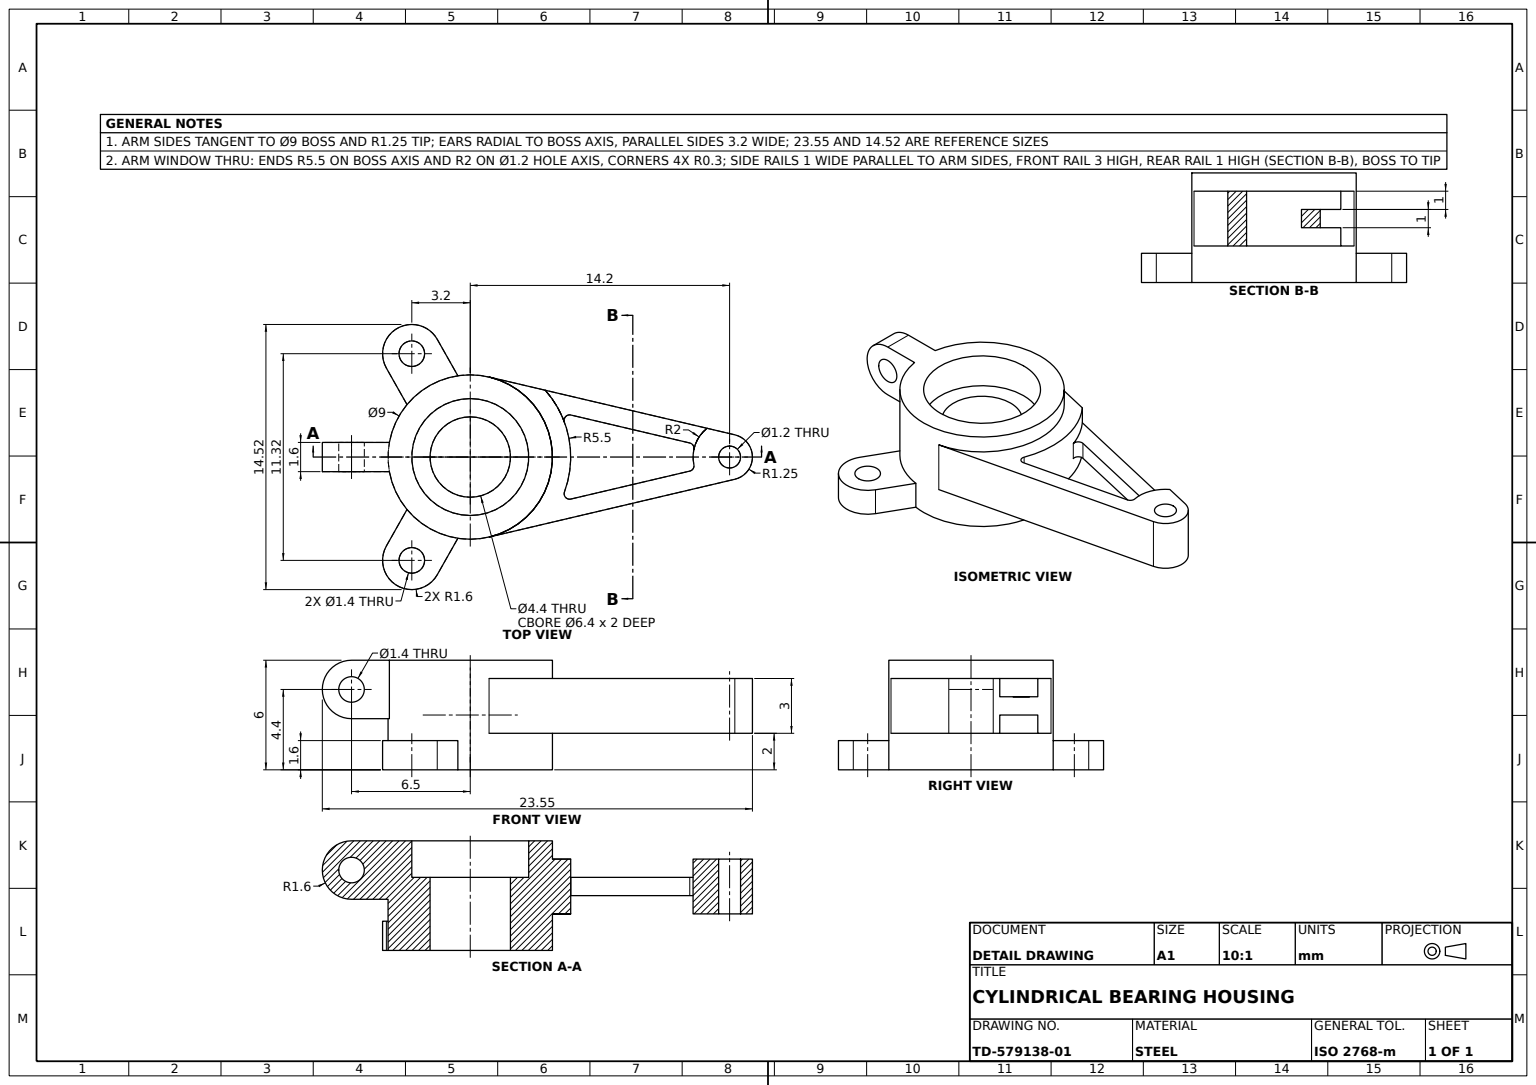
ISO-10303-21;
HEADER;
FILE_DESCRIPTION((''),'2;1');
FILE_NAME('','',(''),(''),'','','');
FILE_SCHEMA(('AUTOMOTIVE_DESIGN'));
ENDSEC;
DATA;
#1=APPLICATION_CONTEXT('');
#2=PRODUCT_CONTEXT('',#1,'mechanical');
#3=PRODUCT('','','',(#2));
#4=PRODUCT_DEFINITION_FORMATION('','',#3);
#5=PRODUCT_DEFINITION_CONTEXT('',#1,'design');
#6=PRODUCT_DEFINITION('','',#4,#5);
#7=PRODUCT_DEFINITION_SHAPE('','',#6);
#8=(LENGTH_UNIT()NAMED_UNIT(*)SI_UNIT(.MILLI.,.METRE.));
#9=(NAMED_UNIT(*)PLANE_ANGLE_UNIT()SI_UNIT($,.RADIAN.));
#10=(NAMED_UNIT(*)SI_UNIT($,.STERADIAN.)SOLID_ANGLE_UNIT());
#11=UNCERTAINTY_MEASURE_WITH_UNIT(LENGTH_MEASURE(1.E-05),#8,'distance_accuracy_value','');
#12=(GEOMETRIC_REPRESENTATION_CONTEXT(3)GLOBAL_UNCERTAINTY_ASSIGNED_CONTEXT((#11))GLOBAL_UNIT_ASSIGNED_CONTEXT((#8,#9,#10))REPRESENTATION_CONTEXT('',''));
#13=CARTESIAN_POINT('',(-3.2,1.6,-6.35773806));
#14=VERTEX_POINT('',#13);
#15=CARTESIAN_POINT('',(-3.2,1.6,-4.95773806));
#16=VERTEX_POINT('',#15);
#17=CARTESIAN_POINT('',(-3.2,1.6,-5.65773806));
#18=DIRECTION('',(0.,-1.,0.));
#19=DIRECTION('',(0.,0.,-1.));
#20=AXIS2_PLACEMENT_3D('',#17,#18,#19);
#21=CIRCLE('',#20,0.7);
#22=EDGE_CURVE('',#14,#16,#21,.T.);
#23=ORIENTED_EDGE('',*,*,#22,.T.);
#24=EDGE_CURVE('',#16,#14,#21,.T.);
#25=ORIENTED_EDGE('',*,*,#24,.T.);
#26=EDGE_LOOP('',(#23,#25));
#27=FACE_BOUND('',#26,.T.);
#28=CARTESIAN_POINT('',(-0.67794665,1.6,-4.44863893));
#29=VERTEX_POINT('',#28);
#30=CARTESIAN_POINT('',(-3.46329462,1.6,-2.87325432));
#31=VERTEX_POINT('',#30);
#32=CARTESIAN_POINT('',(0.,1.6,0.));
#33=DIRECTION('',(0.,1.,0.));
#34=AXIS2_PLACEMENT_3D('',#32,#33,#19);
#35=CIRCLE('',#34,4.5);
#36=EDGE_CURVE('',#29,#31,#35,.T.);
#37=ORIENTED_EDGE('',*,*,#36,.F.);
#38=CARTESIAN_POINT('',(-1.80732602,1.6,-6.44543037));
#39=VERTEX_POINT('',#38);
#40=DIRECTION('',(0.492307692,0.,0.870421241));
#41=VECTOR('',#40,1000.);
#42=LINE('',#28,#41);
#43=EDGE_CURVE('',#39,#29,#42,.T.);
#44=ORIENTED_EDGE('',*,*,#43,.F.);
#45=CARTESIAN_POINT('',(-3.2,1.6,-7.25773806));
#46=VERTEX_POINT('',#45);
#47=DIRECTION('',(0.,0.,1.));
#48=AXIS2_PLACEMENT_3D('',#17,#18,#47);
#49=CIRCLE('',#48,1.6);
#50=EDGE_CURVE('',#46,#39,#49,.T.);
#51=ORIENTED_EDGE('',*,*,#50,.F.);
#52=CARTESIAN_POINT('',(-4.59267398,1.6,-4.87004576));
#53=VERTEX_POINT('',#52);
#54=EDGE_CURVE('',#53,#46,#49,.T.);
#55=ORIENTED_EDGE('',*,*,#54,.F.);
#56=DIRECTION('',(-0.492307692,0.,-0.870421241));
#57=VECTOR('',#56,1000.);
#58=LINE('',#30,#57);
#59=EDGE_CURVE('',#31,#53,#58,.T.);
#60=ORIENTED_EDGE('',*,*,#59,.F.);
#61=EDGE_LOOP('',(#37,#44,#51,#55,#60));
#62=FACE_OUTER_BOUND('',#61,.T.);
#63=AXIS2_PLACEMENT_3D('',#17,#33,#47);
#64=PLANE('',#63);
#65=ADVANCED_FACE('',(#27,#62),#64,.T.);
#66=CARTESIAN_POINT('',(-3.46329462,1.6,2.87325432));
#67=VERTEX_POINT('',#66);
#68=CARTESIAN_POINT('',(-0.67794665,1.6,4.44863893));
#69=VERTEX_POINT('',#68);
#70=EDGE_CURVE('',#67,#69,#35,.T.);
#71=ORIENTED_EDGE('',*,*,#70,.T.);
#72=CARTESIAN_POINT('',(-0.67794665,0.,4.44863893));
#73=VERTEX_POINT('',#72);
#74=VECTOR('',#18,1000.);
#75=LINE('',#68,#74);
#76=EDGE_CURVE('',#69,#73,#75,.T.);
#77=ORIENTED_EDGE('',*,*,#76,.T.);
#78=CARTESIAN_POINT('',(0.,0.,4.5));
#79=VERTEX_POINT('',#78);
#80=CARTESIAN_POINT('',(0.,0.,0.));
#81=AXIS2_PLACEMENT_3D('',#80,#33,#47);
#82=CIRCLE('',#81,4.5);
#83=EDGE_CURVE('',#73,#79,#82,.T.);
#84=ORIENTED_EDGE('',*,*,#83,.T.);
#85=CARTESIAN_POINT('',(0.,6.,4.5));
#86=VERTEX_POINT('',#85);
#87=LINE('',#85,#74);
#88=EDGE_CURVE('',#86,#79,#87,.T.);
#89=ORIENTED_EDGE('',*,*,#88,.F.);
#90=CARTESIAN_POINT('',(-4.42831797,6.,0.8));
#91=VERTEX_POINT('',#90);
#92=CARTESIAN_POINT('',(0.,6.,0.));
#93=AXIS2_PLACEMENT_3D('',#92,#33,#47);
#94=CIRCLE('',#93,4.5);
#95=EDGE_CURVE('',#91,#86,#94,.T.);
#96=ORIENTED_EDGE('',*,*,#95,.F.);
#97=CARTESIAN_POINT('',(-4.42831797,2.8,0.8));
#98=VERTEX_POINT('',#97);
#99=VECTOR('',#33,1000.);
#100=LINE('',#90,#99);
#101=EDGE_CURVE('',#98,#91,#100,.T.);
#102=ORIENTED_EDGE('',*,*,#101,.F.);
#103=CARTESIAN_POINT('',(-4.42831797,2.8,-0.8));
#104=VERTEX_POINT('',#103);
#105=CARTESIAN_POINT('',(0.,2.8,0.));
#106=AXIS2_PLACEMENT_3D('',#105,#33,#47);
#107=CIRCLE('',#106,4.5);
#108=EDGE_CURVE('',#104,#98,#107,.T.);
#109=ORIENTED_EDGE('',*,*,#108,.F.);
#110=CARTESIAN_POINT('',(-4.42831797,6.,-0.8));
#111=VERTEX_POINT('',#110);
#112=LINE('',#110,#74);
#113=EDGE_CURVE('',#111,#104,#112,.T.);
#114=ORIENTED_EDGE('',*,*,#113,.F.);
#115=CARTESIAN_POINT('',(0.,6.,-4.5));
#116=VERTEX_POINT('',#115);
#117=EDGE_CURVE('',#116,#111,#94,.T.);
#118=ORIENTED_EDGE('',*,*,#117,.F.);
#119=CARTESIAN_POINT('',(0.,0.,-4.5));
#120=VERTEX_POINT('',#119);
#121=LINE('',#115,#74);
#122=EDGE_CURVE('',#116,#120,#121,.T.);
#123=ORIENTED_EDGE('',*,*,#122,.T.);
#124=CARTESIAN_POINT('',(-0.67794665,0.,-4.44863893));
#125=VERTEX_POINT('',#124);
#126=EDGE_CURVE('',#120,#125,#82,.T.);
#127=ORIENTED_EDGE('',*,*,#126,.T.);
#128=LINE('',#28,#74);
#129=EDGE_CURVE('',#29,#125,#128,.T.);
#130=ORIENTED_EDGE('',*,*,#129,.F.);
#131=ORIENTED_EDGE('',*,*,#36,.T.);
#132=CARTESIAN_POINT('',(-3.46329462,0.,-2.87325432));
#133=VERTEX_POINT('',#132);
#134=LINE('',#30,#74);
#135=EDGE_CURVE('',#31,#133,#134,.T.);
#136=ORIENTED_EDGE('',*,*,#135,.T.);
#137=CARTESIAN_POINT('',(-3.46329462,0.,2.87325432));
#138=VERTEX_POINT('',#137);
#139=EDGE_CURVE('',#133,#138,#82,.T.);
#140=ORIENTED_EDGE('',*,*,#139,.T.);
#141=LINE('',#66,#74);
#142=EDGE_CURVE('',#67,#138,#141,.T.);
#143=ORIENTED_EDGE('',*,*,#142,.F.);
#144=EDGE_LOOP('',(#71,#77,#84,#89,#96,#102,#109,#114,#118,#123,#127,#130,#131,#136,#140,#143));
#145=FACE_OUTER_BOUND('',#144,.T.);
#146=AXIS2_PLACEMENT_3D('',#92,#18,#19);
#147=CYLINDRICAL_SURFACE('',#146,4.5);
#148=ADVANCED_FACE('',(#145),#147,.T.);
#149=CARTESIAN_POINT('',(14.48609155,2.,1.21682029));
#150=VERTEX_POINT('',#149);
#151=CARTESIAN_POINT('',(14.48609155,2.,-1.21682029));
#152=VERTEX_POINT('',#151);
#153=CARTESIAN_POINT('',(14.2,2.,0.));
#154=AXIS2_PLACEMENT_3D('',#153,#33,#47);
#155=CIRCLE('',#154,1.25);
#156=EDGE_CURVE('',#150,#152,#155,.T.);
#157=ORIENTED_EDGE('',*,*,#156,.F.);
#158=CARTESIAN_POINT('',(1.02992958,2.,4.38055305));
#159=VERTEX_POINT('',#158);
#160=DIRECTION('',(0.973456234,0.,-0.228873239));
#161=VECTOR('',#160,1000.);
#162=LINE('',#158,#161);
#163=EDGE_CURVE('',#159,#150,#162,.T.);
#164=ORIENTED_EDGE('',*,*,#163,.F.);
#165=CARTESIAN_POINT('',(1.02992958,2.,-4.38055305));
#166=VERTEX_POINT('',#165);
#167=CARTESIAN_POINT('',(0.,2.,0.));
#168=AXIS2_PLACEMENT_3D('',#167,#18,#47);
#169=CIRCLE('',#168,4.5);
#170=EDGE_CURVE('',#166,#159,#169,.T.);
#171=ORIENTED_EDGE('',*,*,#170,.F.);
#172=CARTESIAN_POINT('',(4.10826848,2.,-3.65679232));
#173=VERTEX_POINT('',#172);
#174=DIRECTION('',(-0.973456234,0.,-0.228873239));
#175=VECTOR('',#174,1000.);
#176=LINE('',#165,#175);
#177=EDGE_CURVE('',#173,#166,#176,.T.);
#178=ORIENTED_EDGE('',*,*,#177,.F.);
#179=CARTESIAN_POINT('',(5.1598984,2.,1.90406105));
#180=VERTEX_POINT('',#179);
#181=CIRCLE('',#168,5.5);
#182=EDGE_CURVE('',#173,#180,#181,.T.);
#183=ORIENTED_EDGE('',*,*,#182,.T.);
#184=CARTESIAN_POINT('',(5.44134741,2.,2.30791892));
#185=VERTEX_POINT('',#184);
#186=CARTESIAN_POINT('',(5.44134741,2.,2.00791892));
#187=AXIS2_PLACEMENT_3D('',#186,#33,#47);
#188=CIRCLE('',#187,0.3);
#189=EDGE_CURVE('',#180,#185,#188,.T.);
#190=ORIENTED_EDGE('',*,*,#189,.T.);
#191=CARTESIAN_POINT('',(5.51000938,2.,2.29995579));
#192=VERTEX_POINT('',#191);
#193=EDGE_CURVE('',#185,#192,#188,.T.);
#194=ORIENTED_EDGE('',*,*,#193,.T.);
#195=CARTESIAN_POINT('',(12.01879809,2.,0.76964811));
#196=VERTEX_POINT('',#195);
#197=CARTESIAN_POINT('',(0.80105634,2.,3.40709682));
#198=LINE('',#197,#161);
#199=EDGE_CURVE('',#192,#196,#198,.T.);
#200=ORIENTED_EDGE('',*,*,#199,.T.);
#201=CARTESIAN_POINT('',(12.24359662,2.,0.41531412));
#202=VERTEX_POINT('',#201);
#203=CARTESIAN_POINT('',(11.95013611,2.,0.47761124));
#204=AXIS2_PLACEMENT_3D('',#203,#33,#47);
#205=CIRCLE('',#204,0.3);
#206=EDGE_CURVE('',#196,#202,#205,.T.);
#207=ORIENTED_EDGE('',*,*,#206,.T.);
#208=CARTESIAN_POINT('',(12.96628349,2.,-1.57414852));
#209=VERTEX_POINT('',#208);
#210=AXIS2_PLACEMENT_3D('',#153,#18,#47);
#211=CIRCLE('',#210,2.);
#212=EDGE_CURVE('',#202,#209,#211,.T.);
#213=ORIENTED_EDGE('',*,*,#212,.T.);
#214=EDGE_CURVE('',#152,#209,#176,.T.);
#215=ORIENTED_EDGE('',*,*,#214,.F.);
#216=EDGE_LOOP('',(#157,#164,#171,#178,#183,#190,#194,#200,#207,#213,#215));
#217=FACE_OUTER_BOUND('',#216,.T.);
#218=CARTESIAN_POINT('',(14.2,2.,0.6));
#219=VERTEX_POINT('',#218);
#220=CARTESIAN_POINT('',(14.2,2.,-0.6));
#221=VERTEX_POINT('',#220);
#222=CIRCLE('',#154,0.6);
#223=EDGE_CURVE('',#219,#221,#222,.T.);
#224=ORIENTED_EDGE('',*,*,#223,.T.);
#225=EDGE_CURVE('',#221,#219,#222,.T.);
#226=ORIENTED_EDGE('',*,*,#225,.T.);
#227=EDGE_LOOP('',(#224,#226));
#228=FACE_BOUND('',#227,.T.);
#229=AXIS2_PLACEMENT_3D('',#167,#33,#47);
#230=PLANE('',#229);
#231=ADVANCED_FACE('',(#217,#228),#230,.F.);
#232=CARTESIAN_POINT('',(-8.1,4.4,0.8));
#233=VERTEX_POINT('',#232);
#234=CARTESIAN_POINT('',(-8.1,4.4,-0.8));
#235=VERTEX_POINT('',#234);
#236=VECTOR('',#19,1000.);
#237=LINE('',#232,#236);
#238=EDGE_CURVE('',#233,#235,#237,.T.);
#239=ORIENTED_EDGE('',*,*,#238,.T.);
#240=CARTESIAN_POINT('',(-6.5,2.8,-0.8));
#241=VERTEX_POINT('',#240);
#242=CARTESIAN_POINT('',(-6.5,4.4,-0.8));
#243=DIRECTION('',(1.,0.,0.));
#244=AXIS2_PLACEMENT_3D('',#242,#47,#243);
#245=CIRCLE('',#244,1.6);
#246=EDGE_CURVE('',#235,#241,#245,.T.);
#247=ORIENTED_EDGE('',*,*,#246,.T.);
#248=CARTESIAN_POINT('',(-6.5,2.8,0.8));
#249=VERTEX_POINT('',#248);
#250=LINE('',#248,#236);
#251=EDGE_CURVE('',#249,#241,#250,.T.);
#252=ORIENTED_EDGE('',*,*,#251,.F.);
#253=CARTESIAN_POINT('',(-6.5,4.4,0.8));
#254=AXIS2_PLACEMENT_3D('',#253,#47,#243);
#255=CIRCLE('',#254,1.6);
#256=EDGE_CURVE('',#233,#249,#255,.T.);
#257=ORIENTED_EDGE('',*,*,#256,.F.);
#258=EDGE_LOOP('',(#239,#247,#252,#257));
#259=FACE_OUTER_BOUND('',#258,.T.);
#260=DIRECTION('',(-1.,0.,0.));
#261=AXIS2_PLACEMENT_3D('',#253,#19,#260);
#262=CYLINDRICAL_SURFACE('',#261,1.6);
#263=ADVANCED_FACE('',(#259),#262,.T.);
#264=CARTESIAN_POINT('',(-4.59267398,0.,-4.87004576));
#265=VERTEX_POINT('',#264);
#266=CARTESIAN_POINT('',(-3.2,0.,-7.25773806));
#267=VERTEX_POINT('',#266);
#268=CARTESIAN_POINT('',(-3.2,0.,-5.65773806));
#269=AXIS2_PLACEMENT_3D('',#268,#18,#47);
#270=CIRCLE('',#269,1.6);
#271=EDGE_CURVE('',#265,#267,#270,.T.);
#272=ORIENTED_EDGE('',*,*,#271,.F.);
#273=LINE('',#52,#74);
#274=EDGE_CURVE('',#53,#265,#273,.T.);
#275=ORIENTED_EDGE('',*,*,#274,.F.);
#276=ORIENTED_EDGE('',*,*,#54,.T.);
#277=LINE('',#45,#74);
#278=EDGE_CURVE('',#46,#267,#277,.T.);
#279=ORIENTED_EDGE('',*,*,#278,.T.);
#280=EDGE_LOOP('',(#272,#275,#276,#279));
#281=FACE_OUTER_BOUND('',#280,.T.);
#282=CYLINDRICAL_SURFACE('',#20,1.6);
#283=ADVANCED_FACE('',(#281),#282,.T.);
#284=CARTESIAN_POINT('',(0.,6.,3.2));
#285=VERTEX_POINT('',#284);
#286=CARTESIAN_POINT('',(0.,6.,-3.2));
#287=VERTEX_POINT('',#286);
#288=CIRCLE('',#93,3.2);
#289=EDGE_CURVE('',#285,#287,#288,.T.);
#290=ORIENTED_EDGE('',*,*,#289,.T.);
#291=CARTESIAN_POINT('',(0.,4.,-3.2));
#292=VERTEX_POINT('',#291);
#293=LINE('',#286,#99);
#294=EDGE_CURVE('',#292,#287,#293,.T.);
#295=ORIENTED_EDGE('',*,*,#294,.F.);
#296=CARTESIAN_POINT('',(0.,4.,3.2));
#297=VERTEX_POINT('',#296);
#298=CARTESIAN_POINT('',(0.,4.,0.));
#299=AXIS2_PLACEMENT_3D('',#298,#33,#47);
#300=CIRCLE('',#299,3.2);
#301=EDGE_CURVE('',#297,#292,#300,.T.);
#302=ORIENTED_EDGE('',*,*,#301,.F.);
#303=LINE('',#284,#99);
#304=EDGE_CURVE('',#297,#285,#303,.T.);
#305=ORIENTED_EDGE('',*,*,#304,.T.);
#306=EDGE_LOOP('',(#290,#295,#302,#305));
#307=FACE_OUTER_BOUND('',#306,.T.);
#308=CYLINDRICAL_SURFACE('',#93,3.2);
#309=ADVANCED_FACE('',(#307),#308,.F.);
#310=CARTESIAN_POINT('',(-1.80732602,1.6,6.44543037));
#311=VERTEX_POINT('',#310);
#312=CARTESIAN_POINT('',(-1.80732602,0.,6.44543037));
#313=VERTEX_POINT('',#312);
#314=LINE('',#310,#74);
#315=EDGE_CURVE('',#311,#313,#314,.T.);
#316=ORIENTED_EDGE('',*,*,#315,.F.);
#317=CARTESIAN_POINT('',(-4.59267398,1.6,4.87004576));
#318=VERTEX_POINT('',#317);
#319=CARTESIAN_POINT('',(-3.2,1.6,5.65773806));
#320=AXIS2_PLACEMENT_3D('',#319,#18,#19);
#321=CIRCLE('',#320,1.6);
#322=EDGE_CURVE('',#311,#318,#321,.T.);
#323=ORIENTED_EDGE('',*,*,#322,.T.);
#324=CARTESIAN_POINT('',(-4.59267398,0.,4.87004576));
#325=VERTEX_POINT('',#324);
#326=LINE('',#317,#74);
#327=EDGE_CURVE('',#318,#325,#326,.T.);
#328=ORIENTED_EDGE('',*,*,#327,.T.);
#329=CARTESIAN_POINT('',(-3.2,0.,5.65773806));
#330=AXIS2_PLACEMENT_3D('',#329,#18,#19);
#331=CIRCLE('',#330,1.6);
#332=EDGE_CURVE('',#313,#325,#331,.T.);
#333=ORIENTED_EDGE('',*,*,#332,.F.);
#334=EDGE_LOOP('',(#316,#323,#328,#333));
#335=FACE_OUTER_BOUND('',#334,.T.);
#336=CYLINDRICAL_SURFACE('',#320,1.6);
#337=ADVANCED_FACE('',(#335),#336,.T.);
#338=CARTESIAN_POINT('',(-7.2,4.4,0.8));
#339=VERTEX_POINT('',#338);
#340=CARTESIAN_POINT('',(-5.8,4.4,0.8));
#341=VERTEX_POINT('',#340);
#342=CIRCLE('',#254,0.7);
#343=EDGE_CURVE('',#339,#341,#342,.T.);
#344=ORIENTED_EDGE('',*,*,#343,.F.);
#345=EDGE_CURVE('',#341,#339,#342,.T.);
#346=ORIENTED_EDGE('',*,*,#345,.F.);
#347=EDGE_LOOP('',(#344,#346));
#348=FACE_BOUND('',#347,.T.);
#349=ORIENTED_EDGE('',*,*,#256,.T.);
#350=CARTESIAN_POINT('',(-3.7,2.8,0.8));
#351=VECTOR('',#260,1000.);
#352=LINE('',#350,#351);
#353=EDGE_CURVE('',#98,#249,#352,.T.);
#354=ORIENTED_EDGE('',*,*,#353,.F.);
#355=ORIENTED_EDGE('',*,*,#101,.T.);
#356=CARTESIAN_POINT('',(-6.5,6.,0.8));
#357=VERTEX_POINT('',#356);
#358=CARTESIAN_POINT('',(-3.7,6.,0.8));
#359=LINE('',#358,#351);
#360=EDGE_CURVE('',#91,#357,#359,.T.);
#361=ORIENTED_EDGE('',*,*,#360,.T.);
#362=EDGE_CURVE('',#357,#233,#255,.T.);
#363=ORIENTED_EDGE('',*,*,#362,.T.);
#364=EDGE_LOOP('',(#349,#354,#355,#361,#363));
#365=FACE_OUTER_BOUND('',#364,.T.);
#366=AXIS2_PLACEMENT_3D('',#358,#19,#260);
#367=PLANE('',#366);
#368=ADVANCED_FACE('',(#348,#365),#367,.F.);
#369=ORIENTED_EDGE('',*,*,#76,.F.);
#370=DIRECTION('',(-0.492307692,0.,0.870421241));
#371=VECTOR('',#370,1000.);
#372=LINE('',#68,#371);
#373=EDGE_CURVE('',#69,#311,#372,.T.);
#374=ORIENTED_EDGE('',*,*,#373,.T.);
#375=ORIENTED_EDGE('',*,*,#315,.T.);
#376=LINE('',#72,#371);
#377=EDGE_CURVE('',#73,#313,#376,.T.);
#378=ORIENTED_EDGE('',*,*,#377,.F.);
#379=EDGE_LOOP('',(#369,#374,#375,#378));
#380=FACE_OUTER_BOUND('',#379,.T.);
#381=DIRECTION('',(0.870421241,0.,0.492307692));
#382=DIRECTION('',(0.492307692,0.,-0.870421241));
#383=AXIS2_PLACEMENT_3D('',#68,#381,#382);
#384=PLANE('',#383);
#385=ADVANCED_FACE('',(#380),#384,.T.);
#386=CARTESIAN_POINT('',(-5.8,4.4,-0.8));
#387=VERTEX_POINT('',#386);
#388=LINE('',#340,#236);
#389=EDGE_CURVE('',#341,#387,#388,.T.);
#390=ORIENTED_EDGE('',*,*,#389,.T.);
#391=CARTESIAN_POINT('',(-7.2,4.4,-0.8));
#392=VERTEX_POINT('',#391);
#393=CIRCLE('',#244,0.7);
#394=EDGE_CURVE('',#392,#387,#393,.T.);
#395=ORIENTED_EDGE('',*,*,#394,.F.);
#396=LINE('',#338,#236);
#397=EDGE_CURVE('',#339,#392,#396,.T.);
#398=ORIENTED_EDGE('',*,*,#397,.F.);
#399=ORIENTED_EDGE('',*,*,#343,.T.);
#400=EDGE_LOOP('',(#390,#395,#398,#399));
#401=FACE_OUTER_BOUND('',#400,.T.);
#402=CYLINDRICAL_SURFACE('',#261,0.7);
#403=ADVANCED_FACE('',(#401),#402,.F.);
#404=ORIENTED_EDGE('',*,*,#163,.T.);
#405=CARTESIAN_POINT('',(14.48609155,5.,1.21682029));
#406=VERTEX_POINT('',#405);
#407=LINE('',#149,#99);
#408=EDGE_CURVE('',#150,#406,#407,.T.);
#409=ORIENTED_EDGE('',*,*,#408,.T.);
#410=CARTESIAN_POINT('',(1.02992958,5.,4.38055305));
#411=VERTEX_POINT('',#410);
#412=LINE('',#410,#161);
#413=EDGE_CURVE('',#411,#406,#412,.T.);
#414=ORIENTED_EDGE('',*,*,#413,.F.);
#415=LINE('',#158,#99);
#416=EDGE_CURVE('',#159,#411,#415,.T.);
#417=ORIENTED_EDGE('',*,*,#416,.F.);
#418=EDGE_LOOP('',(#404,#409,#414,#417));
#419=FACE_OUTER_BOUND('',#418,.T.);
#420=DIRECTION('',(0.228873239,0.,0.973456234));
#421=AXIS2_PLACEMENT_3D('',#158,#420,#160);
#422=PLANE('',#421);
#423=ADVANCED_FACE('',(#419),#422,.T.);
#424=CARTESIAN_POINT('',(5.1598984,5.,1.90406105));
#425=VERTEX_POINT('',#424);
#426=CARTESIAN_POINT('',(5.1598984,0.,1.90406105));
#427=LINE('',#426,#99);
#428=EDGE_CURVE('',#180,#425,#427,.T.);
#429=ORIENTED_EDGE('',*,*,#428,.F.);
#430=ORIENTED_EDGE('',*,*,#182,.F.);
#431=CARTESIAN_POINT('',(4.10826848,3.,-3.65679232));
#432=VERTEX_POINT('',#431);
#433=LINE('',#431,#74);
#434=EDGE_CURVE('',#432,#173,#433,.T.);
#435=ORIENTED_EDGE('',*,*,#434,.F.);
#436=CARTESIAN_POINT('',(5.1598984,3.,-1.90406105));
#437=VERTEX_POINT('',#436);
#438=CARTESIAN_POINT('',(0.,3.,0.));
#439=AXIS2_PLACEMENT_3D('',#438,#33,#47);
#440=CIRCLE('',#439,5.5);
#441=EDGE_CURVE('',#437,#432,#440,.T.);
#442=ORIENTED_EDGE('',*,*,#441,.F.);
#443=CARTESIAN_POINT('',(5.1598984,4.,-1.90406105));
#444=VERTEX_POINT('',#443);
#445=CARTESIAN_POINT('',(5.1598984,0.,-1.90406105));
#446=LINE('',#445,#99);
#447=EDGE_CURVE('',#437,#444,#446,.T.);
#448=ORIENTED_EDGE('',*,*,#447,.T.);
#449=CARTESIAN_POINT('',(4.10826848,4.,-3.65679232));
#450=VERTEX_POINT('',#449);
#451=AXIS2_PLACEMENT_3D('',#298,#18,#47);
#452=CIRCLE('',#451,5.5);
#453=EDGE_CURVE('',#450,#444,#452,.T.);
#454=ORIENTED_EDGE('',*,*,#453,.F.);
#455=CARTESIAN_POINT('',(4.10826848,5.,-3.65679232));
#456=VERTEX_POINT('',#455);
#457=LINE('',#449,#99);
#458=EDGE_CURVE('',#450,#456,#457,.T.);
#459=ORIENTED_EDGE('',*,*,#458,.T.);
#460=CARTESIAN_POINT('',(0.,5.,0.));
#461=AXIS2_PLACEMENT_3D('',#460,#18,#47);
#462=CIRCLE('',#461,5.5);
#463=EDGE_CURVE('',#456,#425,#462,.T.);
#464=ORIENTED_EDGE('',*,*,#463,.T.);
#465=EDGE_LOOP('',(#429,#430,#435,#442,#448,#454,#459,#464));
#466=FACE_OUTER_BOUND('',#465,.T.);
#467=CYLINDRICAL_SURFACE('',#81,5.5);
#468=ADVANCED_FACE('',(#466),#467,.T.);
#469=CARTESIAN_POINT('',(-3.2,1.6,6.35773806));
#470=VERTEX_POINT('',#469);
#471=CARTESIAN_POINT('',(-3.2,1.6,4.95773806));
#472=VERTEX_POINT('',#471);
#473=CIRCLE('',#320,0.7);
#474=EDGE_CURVE('',#470,#472,#473,.T.);
#475=ORIENTED_EDGE('',*,*,#474,.F.);
#476=CARTESIAN_POINT('',(-3.2,0.,6.35773806));
#477=VERTEX_POINT('',#476);
#478=LINE('',#469,#74);
#479=EDGE_CURVE('',#470,#477,#478,.T.);
#480=ORIENTED_EDGE('',*,*,#479,.T.);
#481=CARTESIAN_POINT('',(-3.2,0.,4.95773806));
#482=VERTEX_POINT('',#481);
#483=CIRCLE('',#330,0.7);
#484=EDGE_CURVE('',#477,#482,#483,.T.);
#485=ORIENTED_EDGE('',*,*,#484,.T.);
#486=LINE('',#471,#74);
#487=EDGE_CURVE('',#472,#482,#486,.T.);
#488=ORIENTED_EDGE('',*,*,#487,.F.);
#489=EDGE_LOOP('',(#475,#480,#485,#488));
#490=FACE_OUTER_BOUND('',#489,.T.);
#491=CYLINDRICAL_SURFACE('',#320,0.7);
#492=ADVANCED_FACE('',(#490),#491,.F.);
#493=CARTESIAN_POINT('',(12.24359662,3.,-0.41531412));
#494=VERTEX_POINT('',#493);
#495=CARTESIAN_POINT('',(12.01879809,3.,-0.76964811));
#496=VERTEX_POINT('',#495);
#497=CARTESIAN_POINT('',(11.95013611,3.,-0.47761124));
#498=AXIS2_PLACEMENT_3D('',#497,#33,#47);
#499=CIRCLE('',#498,0.3);
#500=EDGE_CURVE('',#494,#496,#499,.T.);
#501=ORIENTED_EDGE('',*,*,#500,.T.);
#502=CARTESIAN_POINT('',(5.51000938,3.,-2.29995579));
#503=VERTEX_POINT('',#502);
#504=CARTESIAN_POINT('',(0.80105634,3.,-3.40709682));
#505=DIRECTION('',(0.973456234,0.,0.228873239));
#506=VECTOR('',#505,1000.);
#507=LINE('',#504,#506);
#508=EDGE_CURVE('',#503,#496,#507,.T.);
#509=ORIENTED_EDGE('',*,*,#508,.F.);
#510=CARTESIAN_POINT('',(5.44134741,3.,-2.00791892));
#511=AXIS2_PLACEMENT_3D('',#510,#33,#47);
#512=CIRCLE('',#511,0.3);
#513=EDGE_CURVE('',#503,#437,#512,.T.);
#514=ORIENTED_EDGE('',*,*,#513,.T.);
#515=ORIENTED_EDGE('',*,*,#441,.T.);
#516=CARTESIAN_POINT('',(12.96628349,3.,-1.57414852));
#517=VERTEX_POINT('',#516);
#518=CARTESIAN_POINT('',(1.02992958,3.,-4.38055305));
#519=LINE('',#518,#175);
#520=EDGE_CURVE('',#517,#432,#519,.T.);
#521=ORIENTED_EDGE('',*,*,#520,.F.);
#522=CARTESIAN_POINT('',(14.2,3.,0.));
#523=AXIS2_PLACEMENT_3D('',#522,#33,#47);
#524=CIRCLE('',#523,2.);
#525=EDGE_CURVE('',#517,#494,#524,.T.);
#526=ORIENTED_EDGE('',*,*,#525,.T.);
#527=EDGE_LOOP('',(#501,#509,#514,#515,#521,#526));
#528=FACE_OUTER_BOUND('',#527,.T.);
#529=PLANE('',#498);
#530=ADVANCED_FACE('',(#528),#529,.F.);
#531=CARTESIAN_POINT('',(0.,0.,-2.2));
#532=VERTEX_POINT('',#531);
#533=CARTESIAN_POINT('',(0.,4.,-2.2));
#534=VERTEX_POINT('',#533);
#535=CARTESIAN_POINT('',(0.,6.,-2.2));
#536=LINE('',#535,#99);
#537=EDGE_CURVE('',#532,#534,#536,.T.);
#538=ORIENTED_EDGE('',*,*,#537,.F.);
#539=CARTESIAN_POINT('',(0.,0.,2.2));
#540=VERTEX_POINT('',#539);
#541=CIRCLE('',#81,2.2);
#542=EDGE_CURVE('',#540,#532,#541,.T.);
#543=ORIENTED_EDGE('',*,*,#542,.F.);
#544=CARTESIAN_POINT('',(0.,4.,2.2));
#545=VERTEX_POINT('',#544);
#546=CARTESIAN_POINT('',(0.,6.,2.2));
#547=LINE('',#546,#99);
#548=EDGE_CURVE('',#540,#545,#547,.T.);
#549=ORIENTED_EDGE('',*,*,#548,.T.);
#550=CIRCLE('',#299,2.2);
#551=EDGE_CURVE('',#545,#534,#550,.T.);
#552=ORIENTED_EDGE('',*,*,#551,.T.);
#553=EDGE_LOOP('',(#538,#543,#549,#552));
#554=FACE_OUTER_BOUND('',#553,.T.);
#555=CYLINDRICAL_SURFACE('',#93,2.2);
#556=ADVANCED_FACE('',(#554),#555,.F.);
#557=ORIENTED_EDGE('',*,*,#50,.T.);
#558=CARTESIAN_POINT('',(-1.80732602,0.,-6.44543037));
#559=VERTEX_POINT('',#558);
#560=LINE('',#38,#74);
#561=EDGE_CURVE('',#39,#559,#560,.T.);
#562=ORIENTED_EDGE('',*,*,#561,.T.);
#563=EDGE_CURVE('',#267,#559,#270,.T.);
#564=ORIENTED_EDGE('',*,*,#563,.F.);
#565=ORIENTED_EDGE('',*,*,#278,.F.);
#566=EDGE_LOOP('',(#557,#562,#564,#565));
#567=FACE_OUTER_BOUND('',#566,.T.);
#568=ADVANCED_FACE('',(#567),#282,.T.);
#569=CARTESIAN_POINT('',(14.2,5.,-0.6));
#570=VERTEX_POINT('',#569);
#571=CARTESIAN_POINT('',(14.2,5.,0.6));
#572=VERTEX_POINT('',#571);
#573=CARTESIAN_POINT('',(14.2,5.,0.));
#574=AXIS2_PLACEMENT_3D('',#573,#33,#47);
#575=CIRCLE('',#574,0.6);
#576=EDGE_CURVE('',#570,#572,#575,.T.);
#577=ORIENTED_EDGE('',*,*,#576,.T.);
#578=CARTESIAN_POINT('',(14.2,0.,0.6));
#579=LINE('',#578,#99);
#580=EDGE_CURVE('',#219,#572,#579,.T.);
#581=ORIENTED_EDGE('',*,*,#580,.F.);
#582=ORIENTED_EDGE('',*,*,#225,.F.);
#583=CARTESIAN_POINT('',(14.2,0.,-0.6));
#584=LINE('',#583,#99);
#585=EDGE_CURVE('',#221,#570,#584,.T.);
#586=ORIENTED_EDGE('',*,*,#585,.T.);
#587=EDGE_LOOP('',(#577,#581,#582,#586));
#588=FACE_OUTER_BOUND('',#587,.T.);
#589=CARTESIAN_POINT('',(14.2,0.,0.));
#590=AXIS2_PLACEMENT_3D('',#589,#33,#47);
#591=CYLINDRICAL_SURFACE('',#590,0.6);
#592=ADVANCED_FACE('',(#588),#591,.F.);
#593=CARTESIAN_POINT('',(-3.7,2.8,-0.8));
#594=LINE('',#593,#351);
#595=EDGE_CURVE('',#104,#241,#594,.T.);
#596=ORIENTED_EDGE('',*,*,#595,.F.);
#597=ORIENTED_EDGE('',*,*,#108,.T.);
#598=ORIENTED_EDGE('',*,*,#353,.T.);
#599=ORIENTED_EDGE('',*,*,#251,.T.);
#600=EDGE_LOOP('',(#596,#597,#598,#599));
#601=FACE_OUTER_BOUND('',#600,.T.);
#602=AXIS2_PLACEMENT_3D('',#350,#33,#47);
#603=PLANE('',#602);
#604=ADVANCED_FACE('',(#601),#603,.F.);
#605=ORIENTED_EDGE('',*,*,#193,.F.);
#606=CARTESIAN_POINT('',(5.44134741,5.,2.30791892));
#607=VERTEX_POINT('',#606);
#608=CARTESIAN_POINT('',(5.44134741,0.,2.30791892));
#609=LINE('',#608,#99);
#610=EDGE_CURVE('',#185,#607,#609,.T.);
#611=ORIENTED_EDGE('',*,*,#610,.T.);
#612=CARTESIAN_POINT('',(5.51000938,5.,2.29995579));
#613=VERTEX_POINT('',#612);
#614=CARTESIAN_POINT('',(5.44134741,5.,2.00791892));
#615=AXIS2_PLACEMENT_3D('',#614,#33,#47);
#616=CIRCLE('',#615,0.3);
#617=EDGE_CURVE('',#607,#613,#616,.T.);
#618=ORIENTED_EDGE('',*,*,#617,.T.);
#619=CARTESIAN_POINT('',(5.51000938,0.,2.29995579));
#620=LINE('',#619,#99);
#621=EDGE_CURVE('',#192,#613,#620,.T.);
#622=ORIENTED_EDGE('',*,*,#621,.F.);
#623=EDGE_LOOP('',(#605,#611,#618,#622));
#624=FACE_OUTER_BOUND('',#623,.T.);
#625=CARTESIAN_POINT('',(5.44134741,0.,2.00791892));
#626=AXIS2_PLACEMENT_3D('',#625,#33,#47);
#627=CYLINDRICAL_SURFACE('',#626,0.3);
#628=ADVANCED_FACE('',(#624),#627,.F.);
#629=CARTESIAN_POINT('',(14.48609155,5.,-1.21682029));
#630=VERTEX_POINT('',#629);
#631=LINE('',#151,#99);
#632=EDGE_CURVE('',#152,#630,#631,.T.);
#633=ORIENTED_EDGE('',*,*,#632,.T.);
#634=CIRCLE('',#574,1.25);
#635=EDGE_CURVE('',#406,#630,#634,.T.);
#636=ORIENTED_EDGE('',*,*,#635,.F.);
#637=ORIENTED_EDGE('',*,*,#408,.F.);
#638=ORIENTED_EDGE('',*,*,#156,.T.);
#639=EDGE_LOOP('',(#633,#636,#637,#638));
#640=FACE_OUTER_BOUND('',#639,.T.);
#641=CYLINDRICAL_SURFACE('',#154,1.25);
#642=ADVANCED_FACE('',(#640),#641,.T.);
#643=CARTESIAN_POINT('',(5.51000938,4.,-2.29995579));
#644=VERTEX_POINT('',#643);
#645=CARTESIAN_POINT('',(12.01879809,4.,-0.76964811));
#646=VERTEX_POINT('',#645);
#647=LINE('',#645,#506);
#648=EDGE_CURVE('',#644,#646,#647,.T.);
#649=ORIENTED_EDGE('',*,*,#648,.T.);
#650=CARTESIAN_POINT('',(12.24359662,4.,-0.41531412));
#651=VERTEX_POINT('',#650);
#652=CARTESIAN_POINT('',(11.95013611,4.,-0.47761124));
#653=AXIS2_PLACEMENT_3D('',#652,#18,#47);
#654=CIRCLE('',#653,0.3);
#655=EDGE_CURVE('',#646,#651,#654,.T.);
#656=ORIENTED_EDGE('',*,*,#655,.T.);
#657=CARTESIAN_POINT('',(12.96628349,4.,-1.57414852));
#658=VERTEX_POINT('',#657);
#659=CARTESIAN_POINT('',(14.2,4.,0.));
#660=AXIS2_PLACEMENT_3D('',#659,#18,#47);
#661=CIRCLE('',#660,2.);
#662=EDGE_CURVE('',#651,#658,#661,.T.);
#663=ORIENTED_EDGE('',*,*,#662,.T.);
#664=LINE('',#657,#175);
#665=EDGE_CURVE('',#658,#450,#664,.T.);
#666=ORIENTED_EDGE('',*,*,#665,.T.);
#667=ORIENTED_EDGE('',*,*,#453,.T.);
#668=CARTESIAN_POINT('',(5.44134741,4.,-2.00791892));
#669=AXIS2_PLACEMENT_3D('',#668,#18,#47);
#670=CIRCLE('',#669,0.3);
#671=EDGE_CURVE('',#444,#644,#670,.T.);
#672=ORIENTED_EDGE('',*,*,#671,.T.);
#673=EDGE_LOOP('',(#649,#656,#663,#666,#667,#672));
#674=FACE_OUTER_BOUND('',#673,.T.);
#675=AXIS2_PLACEMENT_3D('',#659,#33,#47);
#676=PLANE('',#675);
#677=ADVANCED_FACE('',(#674),#676,.T.);
#678=ORIENTED_EDGE('',*,*,#551,.F.);
#679=EDGE_CURVE('',#534,#545,#550,.T.);
#680=ORIENTED_EDGE('',*,*,#679,.F.);
#681=EDGE_LOOP('',(#678,#680));
#682=FACE_BOUND('',#681,.T.);
#683=ORIENTED_EDGE('',*,*,#301,.T.);
#684=EDGE_CURVE('',#292,#297,#300,.T.);
#685=ORIENTED_EDGE('',*,*,#684,.T.);
#686=EDGE_LOOP('',(#683,#685));
#687=FACE_OUTER_BOUND('',#686,.T.);
#688=CARTESIAN_POINT('',(2.2,4.,0.));
#689=AXIS2_PLACEMENT_3D('',#688,#18,#19);
#690=PLANE('',#689);
#691=ADVANCED_FACE('',(#682,#687),#690,.F.);
#692=EDGE_CURVE('',#472,#470,#473,.T.);
#693=ORIENTED_EDGE('',*,*,#692,.F.);
#694=ORIENTED_EDGE('',*,*,#487,.T.);
#695=EDGE_CURVE('',#482,#477,#483,.T.);
#696=ORIENTED_EDGE('',*,*,#695,.T.);
#697=ORIENTED_EDGE('',*,*,#479,.F.);
#698=EDGE_LOOP('',(#693,#694,#696,#697));
#699=FACE_OUTER_BOUND('',#698,.T.);
#700=ADVANCED_FACE('',(#699),#491,.F.);
#701=EDGE_CURVE('',#86,#116,#94,.T.);
#702=ORIENTED_EDGE('',*,*,#701,.F.);
#703=ORIENTED_EDGE('',*,*,#88,.T.);
#704=EDGE_CURVE('',#79,#120,#82,.T.);
#705=ORIENTED_EDGE('',*,*,#704,.T.);
#706=ORIENTED_EDGE('',*,*,#122,.F.);
#707=EDGE_LOOP('',(#702,#703,#705,#706));
#708=FACE_OUTER_BOUND('',#707,.T.);
#709=ORIENTED_EDGE('',*,*,#416,.T.);
#710=CARTESIAN_POINT('',(1.02992958,5.,-4.38055305));
#711=VERTEX_POINT('',#710);
#712=CIRCLE('',#461,4.5);
#713=EDGE_CURVE('',#711,#411,#712,.T.);
#714=ORIENTED_EDGE('',*,*,#713,.F.);
#715=LINE('',#165,#99);
#716=EDGE_CURVE('',#166,#711,#715,.T.);
#717=ORIENTED_EDGE('',*,*,#716,.F.);
#718=ORIENTED_EDGE('',*,*,#170,.T.);
#719=EDGE_LOOP('',(#709,#714,#717,#718));
#720=FACE_BOUND('',#719,.T.);
#721=ADVANCED_FACE('',(#708,#720),#147,.T.);
#722=ORIENTED_EDGE('',*,*,#345,.T.);
#723=ORIENTED_EDGE('',*,*,#397,.T.);
#724=EDGE_CURVE('',#387,#392,#393,.T.);
#725=ORIENTED_EDGE('',*,*,#724,.F.);
#726=ORIENTED_EDGE('',*,*,#389,.F.);
#727=EDGE_LOOP('',(#722,#723,#725,#726));
#728=FACE_OUTER_BOUND('',#727,.T.);
#729=ADVANCED_FACE('',(#728),#402,.F.);
#730=ORIENTED_EDGE('',*,*,#632,.F.);
#731=ORIENTED_EDGE('',*,*,#214,.T.);
#732=LINE('',#516,#74);
#733=EDGE_CURVE('',#517,#209,#732,.T.);
#734=ORIENTED_EDGE('',*,*,#733,.F.);
#735=ORIENTED_EDGE('',*,*,#520,.T.);
#736=ORIENTED_EDGE('',*,*,#434,.T.);
#737=ORIENTED_EDGE('',*,*,#177,.T.);
#738=ORIENTED_EDGE('',*,*,#716,.T.);
#739=LINE('',#710,#175);
#740=EDGE_CURVE('',#456,#711,#739,.T.);
#741=ORIENTED_EDGE('',*,*,#740,.F.);
#742=ORIENTED_EDGE('',*,*,#458,.F.);
#743=ORIENTED_EDGE('',*,*,#665,.F.);
#744=CARTESIAN_POINT('',(12.96628349,5.,-1.57414852));
#745=VERTEX_POINT('',#744);
#746=LINE('',#657,#99);
#747=EDGE_CURVE('',#658,#745,#746,.T.);
#748=ORIENTED_EDGE('',*,*,#747,.T.);
#749=EDGE_CURVE('',#630,#745,#739,.T.);
#750=ORIENTED_EDGE('',*,*,#749,.F.);
#751=EDGE_LOOP('',(#730,#731,#734,#735,#736,#737,#738,#741,#742,#743,#748,#750));
#752=FACE_OUTER_BOUND('',#751,.T.);
#753=DIRECTION('',(0.228873239,0.,-0.973456234));
#754=AXIS2_PLACEMENT_3D('',#165,#753,#174);
#755=PLANE('',#754);
#756=ADVANCED_FACE('',(#752),#755,.T.);
#757=ORIENTED_EDGE('',*,*,#377,.T.);
#758=ORIENTED_EDGE('',*,*,#332,.T.);
#759=VECTOR('',#382,1000.);
#760=LINE('',#137,#759);
#761=EDGE_CURVE('',#325,#138,#760,.T.);
#762=ORIENTED_EDGE('',*,*,#761,.T.);
#763=ORIENTED_EDGE('',*,*,#139,.F.);
#764=LINE('',#132,#57);
#765=EDGE_CURVE('',#133,#265,#764,.T.);
#766=ORIENTED_EDGE('',*,*,#765,.T.);
#767=ORIENTED_EDGE('',*,*,#271,.T.);
#768=ORIENTED_EDGE('',*,*,#563,.T.);
#769=LINE('',#124,#41);
#770=EDGE_CURVE('',#559,#125,#769,.T.);
#771=ORIENTED_EDGE('',*,*,#770,.T.);
#772=ORIENTED_EDGE('',*,*,#126,.F.);
#773=ORIENTED_EDGE('',*,*,#704,.F.);
#774=ORIENTED_EDGE('',*,*,#83,.F.);
#775=EDGE_LOOP('',(#757,#758,#762,#763,#766,#767,#768,#771,#772,#773,#774));
#776=FACE_OUTER_BOUND('',#775,.T.);
#777=ORIENTED_EDGE('',*,*,#542,.T.);
#778=EDGE_CURVE('',#532,#540,#541,.T.);
#779=ORIENTED_EDGE('',*,*,#778,.T.);
#780=EDGE_LOOP('',(#777,#779));
#781=FACE_BOUND('',#780,.T.);
#782=ORIENTED_EDGE('',*,*,#695,.F.);
#783=ORIENTED_EDGE('',*,*,#484,.F.);
#784=EDGE_LOOP('',(#782,#783));
#785=FACE_BOUND('',#784,.T.);
#786=CARTESIAN_POINT('',(-3.2,0.,-6.35773806));
#787=VERTEX_POINT('',#786);
#788=CARTESIAN_POINT('',(-3.2,0.,-4.95773806));
#789=VERTEX_POINT('',#788);
#790=AXIS2_PLACEMENT_3D('',#268,#18,#19);
#791=CIRCLE('',#790,0.7);
#792=EDGE_CURVE('',#787,#789,#791,.T.);
#793=ORIENTED_EDGE('',*,*,#792,.F.);
#794=EDGE_CURVE('',#789,#787,#791,.T.);
#795=ORIENTED_EDGE('',*,*,#794,.F.);
#796=EDGE_LOOP('',(#793,#795));
#797=FACE_BOUND('',#796,.T.);
#798=PLANE('',#81);
#799=ADVANCED_FACE('',(#776,#781,#785,#797),#798,.F.);
#800=CARTESIAN_POINT('',(12.01879809,5.,0.76964811));
#801=VERTEX_POINT('',#800);
#802=CARTESIAN_POINT('',(0.80105634,5.,3.40709682));
#803=LINE('',#802,#161);
#804=EDGE_CURVE('',#613,#801,#803,.T.);
#805=ORIENTED_EDGE('',*,*,#804,.T.);
#806=CARTESIAN_POINT('',(12.01879809,0.,0.76964811));
#807=LINE('',#806,#99);
#808=EDGE_CURVE('',#196,#801,#807,.T.);
#809=ORIENTED_EDGE('',*,*,#808,.F.);
#810=ORIENTED_EDGE('',*,*,#199,.F.);
#811=ORIENTED_EDGE('',*,*,#621,.T.);
#812=EDGE_LOOP('',(#805,#809,#810,#811));
#813=FACE_OUTER_BOUND('',#812,.T.);
#814=AXIS2_PLACEMENT_3D('',#619,#420,#160);
#815=PLANE('',#814);
#816=ADVANCED_FACE('',(#813),#815,.F.);
#817=CARTESIAN_POINT('',(12.01879809,0.,-0.76964811));
#818=LINE('',#817,#99);
#819=EDGE_CURVE('',#496,#646,#818,.T.);
#820=ORIENTED_EDGE('',*,*,#819,.F.);
#821=ORIENTED_EDGE('',*,*,#500,.F.);
#822=CARTESIAN_POINT('',(12.24359662,0.,-0.41531412));
#823=LINE('',#822,#99);
#824=EDGE_CURVE('',#494,#651,#823,.T.);
#825=ORIENTED_EDGE('',*,*,#824,.T.);
#826=ORIENTED_EDGE('',*,*,#655,.F.);
#827=EDGE_LOOP('',(#820,#821,#825,#826));
#828=FACE_OUTER_BOUND('',#827,.T.);
#829=CARTESIAN_POINT('',(11.95013611,0.,-0.47761124));
#830=AXIS2_PLACEMENT_3D('',#829,#33,#47);
#831=CYLINDRICAL_SURFACE('',#830,0.3);
#832=ADVANCED_FACE('',(#828),#831,.F.);
#833=ORIENTED_EDGE('',*,*,#513,.F.);
#834=CARTESIAN_POINT('',(5.51000938,0.,-2.29995579));
#835=LINE('',#834,#99);
#836=EDGE_CURVE('',#503,#644,#835,.T.);
#837=ORIENTED_EDGE('',*,*,#836,.T.);
#838=ORIENTED_EDGE('',*,*,#671,.F.);
#839=ORIENTED_EDGE('',*,*,#447,.F.);
#840=EDGE_LOOP('',(#833,#837,#838,#839));
#841=FACE_OUTER_BOUND('',#840,.T.);
#842=CARTESIAN_POINT('',(5.44134741,0.,-2.00791892));
#843=AXIS2_PLACEMENT_3D('',#842,#33,#47);
#844=CYLINDRICAL_SURFACE('',#843,0.3);
#845=ADVANCED_FACE('',(#841),#844,.F.);
#846=ORIENTED_EDGE('',*,*,#327,.F.);
#847=LINE('',#66,#759);
#848=EDGE_CURVE('',#318,#67,#847,.T.);
#849=ORIENTED_EDGE('',*,*,#848,.T.);
#850=ORIENTED_EDGE('',*,*,#142,.T.);
#851=ORIENTED_EDGE('',*,*,#761,.F.);
#852=EDGE_LOOP('',(#846,#849,#850,#851));
#853=FACE_OUTER_BOUND('',#852,.T.);
#854=DIRECTION('',(-0.870421241,0.,-0.492307692));
#855=AXIS2_PLACEMENT_3D('',#66,#854,#370);
#856=PLANE('',#855);
#857=ADVANCED_FACE('',(#853),#856,.T.);
#858=ORIENTED_EDGE('',*,*,#701,.T.);
#859=ORIENTED_EDGE('',*,*,#117,.T.);
#860=CARTESIAN_POINT('',(-6.5,6.,-0.8));
#861=VERTEX_POINT('',#860);
#862=CARTESIAN_POINT('',(-3.7,6.,-0.8));
#863=LINE('',#862,#351);
#864=EDGE_CURVE('',#111,#861,#863,.T.);
#865=ORIENTED_EDGE('',*,*,#864,.T.);
#866=LINE('',#356,#236);
#867=EDGE_CURVE('',#357,#861,#866,.T.);
#868=ORIENTED_EDGE('',*,*,#867,.F.);
#869=ORIENTED_EDGE('',*,*,#360,.F.);
#870=ORIENTED_EDGE('',*,*,#95,.T.);
#871=EDGE_LOOP('',(#858,#859,#865,#868,#869,#870));
#872=FACE_OUTER_BOUND('',#871,.T.);
#873=ORIENTED_EDGE('',*,*,#289,.F.);
#874=EDGE_CURVE('',#287,#285,#288,.T.);
#875=ORIENTED_EDGE('',*,*,#874,.F.);
#876=EDGE_LOOP('',(#873,#875));
#877=FACE_BOUND('',#876,.T.);
#878=PLANE('',#93);
#879=ADVANCED_FACE('',(#872,#877),#878,.T.);
#880=ORIENTED_EDGE('',*,*,#537,.T.);
#881=ORIENTED_EDGE('',*,*,#679,.T.);
#882=ORIENTED_EDGE('',*,*,#548,.F.);
#883=ORIENTED_EDGE('',*,*,#778,.F.);
#884=EDGE_LOOP('',(#880,#881,#882,#883));
#885=FACE_OUTER_BOUND('',#884,.T.);
#886=ADVANCED_FACE('',(#885),#555,.F.);
#887=ORIENTED_EDGE('',*,*,#294,.T.);
#888=ORIENTED_EDGE('',*,*,#874,.T.);
#889=ORIENTED_EDGE('',*,*,#304,.F.);
#890=ORIENTED_EDGE('',*,*,#684,.F.);
#891=EDGE_LOOP('',(#887,#888,#889,#890));
#892=FACE_OUTER_BOUND('',#891,.T.);
#893=ADVANCED_FACE('',(#892),#308,.F.);
#894=ORIENTED_EDGE('',*,*,#189,.F.);
#895=ORIENTED_EDGE('',*,*,#428,.T.);
#896=EDGE_CURVE('',#425,#607,#616,.T.);
#897=ORIENTED_EDGE('',*,*,#896,.T.);
#898=ORIENTED_EDGE('',*,*,#610,.F.);
#899=EDGE_LOOP('',(#894,#895,#897,#898));
#900=FACE_OUTER_BOUND('',#899,.T.);
#901=ADVANCED_FACE('',(#900),#627,.F.);
#902=ORIENTED_EDGE('',*,*,#794,.T.);
#903=LINE('',#13,#74);
#904=EDGE_CURVE('',#14,#787,#903,.T.);
#905=ORIENTED_EDGE('',*,*,#904,.F.);
#906=ORIENTED_EDGE('',*,*,#24,.F.);
#907=LINE('',#15,#74);
#908=EDGE_CURVE('',#16,#789,#907,.T.);
#909=ORIENTED_EDGE('',*,*,#908,.T.);
#910=EDGE_LOOP('',(#902,#905,#906,#909));
#911=FACE_OUTER_BOUND('',#910,.T.);
#912=CYLINDRICAL_SURFACE('',#20,0.7);
#913=ADVANCED_FACE('',(#911),#912,.F.);
#914=CARTESIAN_POINT('',(12.24359662,5.,0.41531412));
#915=VERTEX_POINT('',#914);
#916=CARTESIAN_POINT('',(12.24359662,0.,0.41531412));
#917=LINE('',#916,#99);
#918=EDGE_CURVE('',#202,#915,#917,.T.);
#919=ORIENTED_EDGE('',*,*,#918,.F.);
#920=ORIENTED_EDGE('',*,*,#206,.F.);
#921=ORIENTED_EDGE('',*,*,#808,.T.);
#922=CARTESIAN_POINT('',(11.95013611,5.,0.47761124));
#923=AXIS2_PLACEMENT_3D('',#922,#33,#47);
#924=CIRCLE('',#923,0.3);
#925=EDGE_CURVE('',#801,#915,#924,.T.);
#926=ORIENTED_EDGE('',*,*,#925,.T.);
#927=EDGE_LOOP('',(#919,#920,#921,#926));
#928=FACE_OUTER_BOUND('',#927,.T.);
#929=CARTESIAN_POINT('',(11.95013611,0.,0.47761124));
#930=AXIS2_PLACEMENT_3D('',#929,#33,#47);
#931=CYLINDRICAL_SURFACE('',#930,0.3);
#932=ADVANCED_FACE('',(#928),#931,.F.);
#933=ORIENTED_EDGE('',*,*,#113,.T.);
#934=ORIENTED_EDGE('',*,*,#595,.T.);
#935=ORIENTED_EDGE('',*,*,#246,.F.);
#936=EDGE_CURVE('',#861,#235,#245,.T.);
#937=ORIENTED_EDGE('',*,*,#936,.F.);
#938=ORIENTED_EDGE('',*,*,#864,.F.);
#939=EDGE_LOOP('',(#933,#934,#935,#937,#938));
#940=FACE_OUTER_BOUND('',#939,.T.);
#941=ORIENTED_EDGE('',*,*,#724,.T.);
#942=ORIENTED_EDGE('',*,*,#394,.T.);
#943=EDGE_LOOP('',(#941,#942));
#944=FACE_BOUND('',#943,.T.);
#945=AXIS2_PLACEMENT_3D('',#593,#47,#243);
#946=PLANE('',#945);
#947=ADVANCED_FACE('',(#940,#944),#946,.F.);
#948=ORIENTED_EDGE('',*,*,#223,.F.);
#949=ORIENTED_EDGE('',*,*,#580,.T.);
#950=EDGE_CURVE('',#572,#570,#575,.T.);
#951=ORIENTED_EDGE('',*,*,#950,.T.);
#952=ORIENTED_EDGE('',*,*,#585,.F.);
#953=EDGE_LOOP('',(#948,#949,#951,#952));
#954=FACE_OUTER_BOUND('',#953,.T.);
#955=ADVANCED_FACE('',(#954),#591,.F.);
#956=ORIENTED_EDGE('',*,*,#765,.F.);
#957=ORIENTED_EDGE('',*,*,#135,.F.);
#958=ORIENTED_EDGE('',*,*,#59,.T.);
#959=ORIENTED_EDGE('',*,*,#274,.T.);
#960=EDGE_LOOP('',(#956,#957,#958,#959));
#961=FACE_OUTER_BOUND('',#960,.T.);
#962=DIRECTION('',(-0.870421241,0.,0.492307692));
#963=AXIS2_PLACEMENT_3D('',#30,#962,#40);
#964=PLANE('',#963);
#965=ADVANCED_FACE('',(#961),#964,.T.);
#966=ORIENTED_EDGE('',*,*,#692,.T.);
#967=ORIENTED_EDGE('',*,*,#474,.T.);
#968=EDGE_LOOP('',(#966,#967));
#969=FACE_BOUND('',#968,.T.);
#970=ORIENTED_EDGE('',*,*,#322,.F.);
#971=ORIENTED_EDGE('',*,*,#373,.F.);
#972=ORIENTED_EDGE('',*,*,#70,.F.);
#973=ORIENTED_EDGE('',*,*,#848,.F.);
#974=EDGE_LOOP('',(#970,#971,#972,#973));
#975=FACE_OUTER_BOUND('',#974,.T.);
#976=PLANE('',#320);
#977=ADVANCED_FACE('',(#969,#975),#976,.F.);
#978=ORIENTED_EDGE('',*,*,#525,.F.);
#979=ORIENTED_EDGE('',*,*,#733,.T.);
#980=ORIENTED_EDGE('',*,*,#212,.F.);
#981=ORIENTED_EDGE('',*,*,#918,.T.);
#982=AXIS2_PLACEMENT_3D('',#573,#18,#47);
#983=CIRCLE('',#982,2.);
#984=EDGE_CURVE('',#915,#745,#983,.T.);
#985=ORIENTED_EDGE('',*,*,#984,.T.);
#986=ORIENTED_EDGE('',*,*,#747,.F.);
#987=ORIENTED_EDGE('',*,*,#662,.F.);
#988=ORIENTED_EDGE('',*,*,#824,.F.);
#989=EDGE_LOOP('',(#978,#979,#980,#981,#985,#986,#987,#988));
#990=FACE_OUTER_BOUND('',#989,.T.);
#991=CYLINDRICAL_SURFACE('',#590,2.);
#992=ADVANCED_FACE('',(#990),#991,.T.);
#993=ORIENTED_EDGE('',*,*,#770,.F.);
#994=ORIENTED_EDGE('',*,*,#561,.F.);
#995=ORIENTED_EDGE('',*,*,#43,.T.);
#996=ORIENTED_EDGE('',*,*,#129,.T.);
#997=EDGE_LOOP('',(#993,#994,#995,#996));
#998=FACE_OUTER_BOUND('',#997,.T.);
#999=DIRECTION('',(0.870421241,0.,-0.492307692));
#1000=AXIS2_PLACEMENT_3D('',#28,#999,#56);
#1001=PLANE('',#1000);
#1002=ADVANCED_FACE('',(#998),#1001,.T.);
#1003=ORIENTED_EDGE('',*,*,#936,.T.);
#1004=ORIENTED_EDGE('',*,*,#238,.F.);
#1005=ORIENTED_EDGE('',*,*,#362,.F.);
#1006=ORIENTED_EDGE('',*,*,#867,.T.);
#1007=EDGE_LOOP('',(#1003,#1004,#1005,#1006));
#1008=FACE_OUTER_BOUND('',#1007,.T.);
#1009=ADVANCED_FACE('',(#1008),#262,.T.);
#1010=ORIENTED_EDGE('',*,*,#819,.T.);
#1011=ORIENTED_EDGE('',*,*,#648,.F.);
#1012=ORIENTED_EDGE('',*,*,#836,.F.);
#1013=ORIENTED_EDGE('',*,*,#508,.T.);
#1014=EDGE_LOOP('',(#1010,#1011,#1012,#1013));
#1015=FACE_OUTER_BOUND('',#1014,.T.);
#1016=AXIS2_PLACEMENT_3D('',#817,#753,#174);
#1017=PLANE('',#1016);
#1018=ADVANCED_FACE('',(#1015),#1017,.F.);
#1019=ORIENTED_EDGE('',*,*,#576,.F.);
#1020=ORIENTED_EDGE('',*,*,#950,.F.);
#1021=EDGE_LOOP('',(#1019,#1020));
#1022=FACE_BOUND('',#1021,.T.);
#1023=ORIENTED_EDGE('',*,*,#896,.F.);
#1024=ORIENTED_EDGE('',*,*,#463,.F.);
#1025=ORIENTED_EDGE('',*,*,#740,.T.);
#1026=ORIENTED_EDGE('',*,*,#713,.T.);
#1027=ORIENTED_EDGE('',*,*,#413,.T.);
#1028=ORIENTED_EDGE('',*,*,#635,.T.);
#1029=ORIENTED_EDGE('',*,*,#749,.T.);
#1030=ORIENTED_EDGE('',*,*,#984,.F.);
#1031=ORIENTED_EDGE('',*,*,#925,.F.);
#1032=ORIENTED_EDGE('',*,*,#804,.F.);
#1033=ORIENTED_EDGE('',*,*,#617,.F.);
#1034=EDGE_LOOP('',(#1023,#1024,#1025,#1026,#1027,#1028,#1029,#1030,#1031,#1032,#1033));
#1035=FACE_OUTER_BOUND('',#1034,.T.);
#1036=AXIS2_PLACEMENT_3D('',#460,#33,#47);
#1037=PLANE('',#1036);
#1038=ADVANCED_FACE('',(#1022,#1035),#1037,.T.);
#1039=ORIENTED_EDGE('',*,*,#904,.T.);
#1040=ORIENTED_EDGE('',*,*,#792,.T.);
#1041=ORIENTED_EDGE('',*,*,#908,.F.);
#1042=ORIENTED_EDGE('',*,*,#22,.F.);
#1043=EDGE_LOOP('',(#1039,#1040,#1041,#1042));
#1044=FACE_OUTER_BOUND('',#1043,.T.);
#1045=ADVANCED_FACE('',(#1044),#912,.F.);
#1046=CLOSED_SHELL('',(#65,#148,#231,#263,#283,#309,#337,#368,#385,#403,#423,#468,#492,#530,#556,#568,#592,#604,#628,#642,#677,#691,#700,#721,#729,#756,#799,#816,#832,#845,#857,#879,#886,#893,#901,#913,#932,#947,#955,#965,#977,#992,#1002,#1009,#1018,#1038,#1045));
#1047=MANIFOLD_SOLID_BREP('',#1046);
#1048=ADVANCED_BREP_SHAPE_REPRESENTATION('',(#1047),#12);
#1049=SHAPE_DEFINITION_REPRESENTATION(#7,#1048);
ENDSEC;
END-ISO-10303-21;
